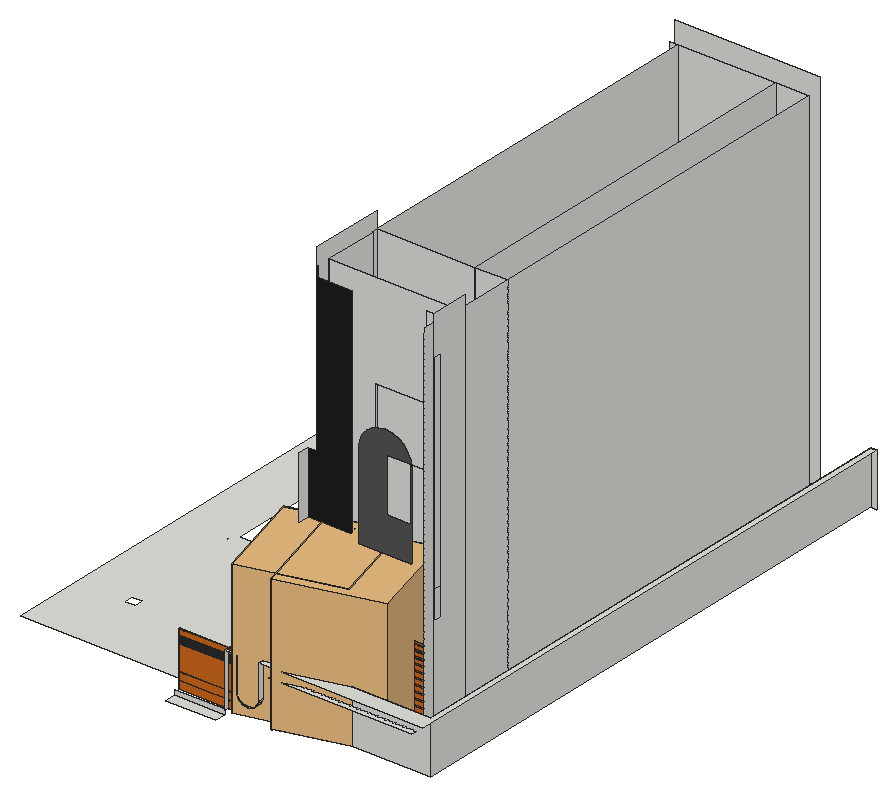
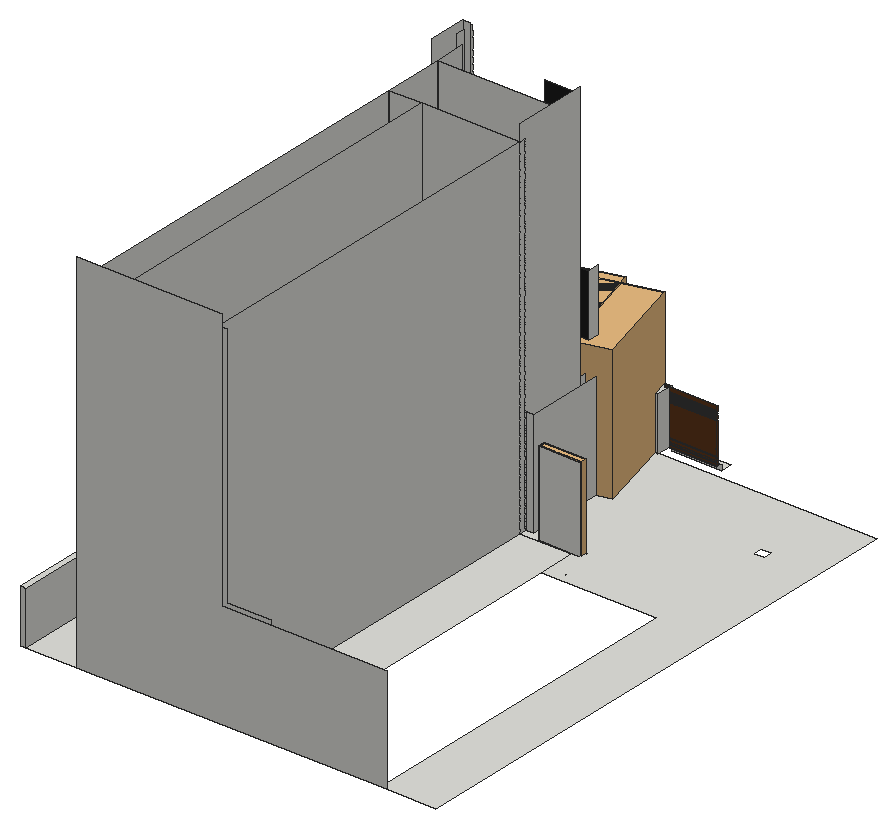
# SketchUp Ruby script. Lengths in inches.
U = 1.inch
M = Sketchup.active_model
def pt(a) = Geom::Point3d.new(a.map { |v| v * U })
def face(e, loops, mat)
  f = e.add_face(loops[0].map { |a| pt(a) })
  loops[1..].each { |l| e.add_face(l.map { |a| pt(a) }).erase! }
  f.material = f.back_material = mat if mat
  f
end
# faces: each face lists its corners as indices into pts; further lists are holes
def faces(e, pts, list, mat = nil) = list.each { |f| face(e, (f[0].is_a?(Array) ? f : [f]).map { |l| l.map { |i| pts[i] } }, mat) }
# xy, xz, yz: faces in a plane at the given z, y or x. An outline is a flat list of corners, or four numbers for a rectangle; further outlines are holes
def ring(l) = l.size == 4 ? [[l[0], l[1]], [l[2], l[1]], [l[2], l[3]], [l[0], l[3]]] : l.each_slice(2).to_a
def flat(e, list, mat, &to3) = list.each { |f| face(e, (f[0].is_a?(Array) ? f : [f]).map { |l| ring(l).map { |u, v| to3.(u, v) } }, mat) }
def xy(e, z, list, mat = nil) = flat(e, list, mat) { |x, y| [x, y, z] }
def xz(e, y, list, mat = nil) = flat(e, list, mat) { |x, z| [x, y, z] }
def yz(e, x, list, mat = nil) = flat(e, list, mat) { |y, z| [x, y, z] }
def lines(e, pts, list) = list.each { |a, b| e.add_line(pt(pts[a]), pt(pts[b])) }
# prism: a flat outline (further loops are holes) pulled along v
def prism(e, loops, v, mat = nil)
  f = face(e, loops, mat); d = Geom::Vector3d.new(v.map { |x| x * U })
  f.pushpull(f.normal.samedirection?(d) ? d.length : -d.length)
end
def box(e, o, s, mat = nil) = prism(e, [[o, [o[0] + s[0], o[1], o[2]], [o[0] + s[0], o[1] + s[1], o[2]], [o[0], o[1] + s[1], o[2]]]], [0, 0, s[2]], mat)
def at(x, y, z, deg = 0) = Geom::Transformation.translation(pt([x, y, z])) * Geom::Transformation.rotation(ORIGIN, Z_AXIS, deg.degrees)
def axes(o, x, y, z) = Geom::Transformation.new([*x, 0, *y, 0, *z, 0, *pt(o).to_a, 1])
def part(name) = M.definitions.add(name)
# library, detail: a bought-in or finely detailed component or shape, given as its bounding box
def library(name, o, s) = part(name).tap { |d| box(d.entities, o, s) }
def detail(e, o, s) = box(e.add_group.entities, o, s)
def put(e, d, t, mat = nil) = e.add_instance(d, t).tap { |i| i.material = mat if mat }
def group(e, t, mat = nil) = e.add_group.tap { |g| g.transformation = t; g.material = mat if mat }.entities
root = M.entities
M.materials.add("[0041_Chocolate]").color = [210, 105, 30]
M.materials.add("[Color M06]").color = [84, 84, 84]
M.materials.add("[Color M08]").color = [30, 30, 30]
M.materials.add("[Wood Veneer 01]2").color = [94, 55, 29]
c1 = library("元件\#5",[-4.39,0,0],[5.37,35.83,90.55])
c2 = part("Slatted screen panel")
xy(c2.entities,0,[[0,0,255.91,1.97]],"[Wood Veneer 01]2")
xy(c2.entities,16.54,[[0,1.18,255.91,1.97]],"[Wood Veneer 01]2")
xy(c2.entities,16.93,[[0,0,255.91,1.18]],"[Wood Veneer 01]2")
xy(c2.entities,17.78,[[0,0,255.91,1.18]],"[Wood Veneer 01]2")
xy(c2.entities,34.45,[[0,0,255.91,1.18]],"[Wood Veneer 01]2")
xy(c2.entities,35.07,[[0,0,255.91,1.18]],"[Wood Veneer 01]2")
xy(c2.entities,89.37,[[0,0,255.91,1.97]],"[Wood Veneer 01]2")
xy(c2.entities,92.91,[[0,0,255.91,1.97]],"[Wood Veneer 01]2")
xy(c2.entities,94.49,[[0,0,255.91,1.97]],"[Wood Veneer 01]2")
xy(c2.entities,97.64,[[0,0,255.91,1.97]],"[Wood Veneer 01]2")
xy(c2.entities,99.21,[[0,0,255.91,1.97]],"[Wood Veneer 01]2")
xy(c2.entities,102.36,[[0,0,255.91,1.97]],"[Wood Veneer 01]2")
xy(c2.entities,103.9375,[[0,0,255.91,1.97]],"[Wood Veneer 01]2")
xy(c2.entities,107.48,[[0,0,255.91,1.97]],"[Wood Veneer 01]2")
xy(c2.entities,119.29,[[0,0,255.91,1.97]],"[Wood Veneer 01]2")
xz(c2.entities,0,[[0,0,255.91,16.93],[0,17.78,255.91,34.45],[0,35.07,255.91,89.37],[0,92.91,255.91,94.49],[0,97.64,255.91,99.21],
  [0,102.36,255.91,103.9375],[0,107.48,255.91,119.29]],"[0041_Chocolate]")
xz(c2.entities,1.18,[[0,16.54,255.91,16.93],[0,16.93,255.91,17.78],[0,34.45,255.91,35.07]],"[Wood Veneer 01]2")
xz(c2.entities,1.97,[[0,0,255.91,1.57],[0,1.57,255.91,5.51],[0,5.51,255.91,7.09],[0,7.09,255.91,11.8125],[0,11.8125,255.91,16.54],
  [0,16.54,255.91,19.69],[0,19.69,255.91,89.37],[0,92.91,255.91,94.49],[0,97.64,255.91,99.21],[0,102.36,255.91,103.9375],
  [0,107.48,255.91,109.84],[0,109.84,255.91,119.29]],"[Wood Veneer 01]2")
yz(c2.entities,0,[[0,0,1.97,1.57],[0,1.57,1.97,5.51],[0,5.51,1.97,7.09],[0,7.09,1.97,11.8125],[0,11.8125,0,16.93,1.18,16.93,1.18,16.54,1.97,16.54,1.97,11.8125],
  [1.18,16.54,1.97,19.69],[0,17.78,0,34.45,1.18,34.45,1.18,35.07,0,35.07,0,89.37,1.97,89.37,1.97,19.69,1.18,19.69,1.18,17.78],[0,92.91,1.97,94.49],[0,97.64,1.97,99.21],[0,102.36,1.97,103.9375],
  [0,107.48,1.97,109.84],[0,109.84,1.97,119.29]],"[Wood Veneer 01]2")
yz(c2.entities,255.91,[[0,0,1.97,1.57],[0,1.57,1.97,5.51],[0,5.51,1.97,7.09],[0,7.09,1.97,11.8125],[0,11.8125,1.97,11.8125,1.97,16.54,1.18,16.54,1.18,16.93,0,16.93],
  [1.18,16.54,1.97,19.69],[0,17.78,1.18,17.78,1.18,19.69,1.97,19.69,1.97,89.37,0,89.37,0,35.07,1.18,35.07,1.18,34.45,0,34.45],[0,92.91,1.97,94.49],[0,97.64,1.97,99.21],[0,102.36,1.97,103.9375],
  [0,107.48,1.97,109.84],[0,109.84,1.97,119.29]],"[Wood Veneer 01]2")
p = [[255.91,1.97,103.9375],[255.91,1.97,107.48],[0,1.97,107.48],[0,1.97,103.9375],[0,1.97,92.91],[0,1.97,89.37],
  [255.91,1.97,99.21],[255.91,1.97,102.36],[255.91,1.97,89.37],[255.91,1.97,92.91],[0,1.97,97.64],[0,1.97,94.49],
  [0,1.97,102.36],[0,1.97,99.21],[255.91,1.97,94.49],[255.91,1.97,97.64],[240.94,0,5.51],[240.94,1.97,5.51]]
lines(c2.entities,p,[[0,1],[2,3],[4,5],[6,7],[8,9],[10,11],[12,13],[14,15],[16,17]])
c3 = library("Palm tree",[-4.09,-4.52,0],[193.52,193.51,258.93])
c4 = part("Palm+Tree")
put(c4.entities,c3,at(25.51,-21.81,0,15))
xy(root,0.73,[[2083.4,185.9375,2140.42,198.625]])
xy(root,6.125,[[[1894.57,217.125,2357.5,217.125,2357.5,838.14,1949.9,838.14,1949.9,439.98,2068.38,439.98,2068.38,397.86,2078.42,397.86,2078.42,405.05,2125.61,405.05,2125.61,397.86,2145.53,397.86,2145.53,406.38,2087.21,406.38,2087.21,448.51,1957.13,448.51,1957.13,830.91,2293.73,830.91,2293.73,336.27,2300.52,336.27,2300.52,292.45,2299.64,292.45,2299.64,280.47,2198.21,280.47,2198.21,292.45,2197.71,292.45,2197.71,305.58,2148.59,305.58,2148.59,292.45,2137,292.45,2137,397.86,2125.61,397.86,2125.61,405.05,2078.42,405.05,2078.42,397.86,2068.38,397.86,2068.38,439.98,1949.9,439.98,1949.9,838.14,1894.57,838.14],[1949.9,294.33,1962.9,305.58]],[2198.21,280.47,2293.73,280.47,2293.73,292.45,2292.85,292.45,2292.85,302.0625,2198.21,302.0625],[2293.73,280.47,2299.64,292.45],[2137,292.45,2148.59,305.58],[2197.71,292.45,2198.21,302.46],
  [2292.85,292.45,2293.73,302.46],[2293.73,292.45,2300.52,302.46],[2198.21,302.0625,2292.85,302.46],[[2198.21,302.46,2293.73,302.46,2293.73,406.38,2145.53,406.38,2145.53,397.86,2137,397.86,2137,305.58,2148.59,305.58,2148.59,312.8125,2158.24,312.8125,2158.24,305.58,2198.21,305.58],[2145.53,321.34,2146.71,397.86]],[2198.21,302.46,2198.21,305.58,2158.24,305.58,2158.24,312.8125,2146.71,312.8125,2146.71,336.27,2293.73,336.27,2293.73,302.46],
  [2198.21,302.46,2198.21,305.58,2158.24,305.58,2158.24,312.8125,2198.21,312.8125,2198.21,305.58,2293.73,305.58,2293.73,302.46],[2197.71,302.46,2198.21,305.58],[2293.73,302.46,2300.52,305.58],[2137,305.58,2148.59,312.8125],[2198.21,305.58,2198.21,312.8125,2146.71,312.8125,2146.71,336.27,2293.73,336.27,2293.73,305.58],
  [2148.59,305.58,2158.24,312.8125],[2293.73,305.58,2300.52,336.27],[2137,312.8125,2137,397.86,2145.53,397.86,2145.53,321.34,2146.71,321.34,2146.71,312.8125],[2145.53,321.34,2146.71,397.86],[2146.71,336.27,2293.73,337.5625],
  [2146.71,337.5625,2293.73,337.5625,2293.73,406.38,2145.53,406.38,2145.53,399.07,2146.71,399.07],[2145.53,397.86,2146.71,399.07],[2087.21,406.38,2145.53,830.91],[2145.53,406.38,2256.73,830.91],[2256.73,406.38,2293.73,830.91]])
xy(root,11.08,[[2198.21,280.47,2299.64,281.47]],"[0041_Chocolate]")
xy(root,13.1875,[[2198.21,280.47,2299.64,281.47]],"[0041_Chocolate]")
xy(root,18.14,[[2198.21,280.47,2299.64,281.47]],"[0041_Chocolate]")
xy(root,20.25,[[2198.21,280.47,2299.64,281.47]],"[0041_Chocolate]")
xy(root,25.2,[[2198.21,280.47,2299.64,281.47]],"[0041_Chocolate]")
xy(root,27.3125,[[2198.21,280.47,2299.64,281.47]],"[0041_Chocolate]")
xy(root,32.27,[[2198.21,280.47,2299.64,281.47]],"[0041_Chocolate]")
xy(root,34.375,[[2198.21,280.47,2299.64,281.47]],"[0041_Chocolate]")
xy(root,39.33,[[2198.21,280.47,2299.64,281.47]],"[0041_Chocolate]")
xy(root,41.4375,[[2198.21,280.47,2299.64,281.47]],"[0041_Chocolate]")
xy(root,46.39,[[2198.21,280.47,2299.64,281.47]],"[0041_Chocolate]")
xy(root,48.5,[[2198.21,280.47,2299.64,281.47]],"[0041_Chocolate]")
xy(root,53.45,[[2198.21,280.47,2299.64,281.47]],"[0041_Chocolate]")
xy(root,55.1875,[[2189.5,198.625,2189.5,203.875,2191.125,203.875,2191.125,204.875,2191.875,204.875,2191.875,203.875,2195.125,203.875,2195.125,204.875,2195.875,204.875,2195.875,203.875,2199.125,203.875,2199.125,204.875,2199.875,204.875,2199.875,203.875,2203.125,203.875,2203.125,204.875,2203.875,204.875,2203.875,203.875,2207.125,203.875,2207.125,204.875,2207.875,204.875,2207.875,203.875,2211.125,203.875,2211.125,204.875,2211.875,204.875,2211.875,203.875,2215.125,203.875,2215.125,204.875,2215.875,204.875,2215.875,203.875,2219.125,203.875,2219.125,204.875,2219.875,204.875,2219.875,203.875,2223.125,203.875,2223.125,204.875,2223.875,204.875,2223.875,203.875,2227.125,203.875,2227.125,204.875,2227.875,204.875,2227.875,203.875,2231.125,203.875,2231.125,204.875,2231.875,204.875,2231.875,203.875,2235.125,203.875,2235.125,204.875,2235.875,204.875,2235.875,203.875,2239.125,203.875,2239.125,204.875,2239.875,204.875,2239.875,203.875,2243.125,203.875,2243.125,204.875,2243.875,204.875,2243.875,203.875,2247.125,203.875,2247.125,204.875,2247.875,204.875,2247.875,203.875,2251.125,203.875,2251.125,204.875,2251.875,204.875,2251.875,203.875,2255.125,203.875,2255.125,204.875,2255.875,204.875,2255.875,203.875,2259.125,203.875,2259.125,204.875,2259.875,204.875,2259.875,203.875,2263.125,203.875,2263.125,204.875,2263.875,204.875,2263.875,203.875,2267.125,203.875,2267.125,204.875,2267.875,204.875,2267.875,203.875,2271.125,203.875,2271.125,204.875,2271.875,204.875,2271.875,203.875,2275.125,203.875,2275.125,204.875,2275.875,204.875,2275.875,203.875,2279.125,203.875,2279.125,204.875,2279.875,204.875,2279.875,203.875,2283.125,203.875,2283.125,204.875,2283.875,204.875,2283.875,203.875,2287.125,203.875,2287.125,204.875,2287.875,204.875,2287.875,203.875,2291.125,203.875,2291.125,204.875,2291.875,204.875,2291.875,203.875,2295.125,203.875,2295.125,204.875,2295.875,204.875,2295.875,203.875,2299.125,203.875,2299.125,204.875,2299.875,204.875,2299.875,203.875,2303.125,203.875,2303.125,204.875,2303.875,204.875,2303.875,203.875,2307.125,203.875,2307.125,204.875,2307.875,204.875,2307.875,203.875,2311.125,203.875,2311.125,204.875,2311.875,204.875,2311.875,203.875,2315.125,203.875,2315.125,204.875,2315.875,204.875,2315.875,203.875,2319.125,203.875,2319.125,204.875,2319.875,204.875,2319.875,203.875,2323.125,203.875,2323.125,204.875,2323.875,204.875,2323.875,203.875,2327.125,203.875,2327.125,204.875,2327.875,204.875,2327.875,203.875,2331.125,203.875,2331.125,204.875,2331.875,204.875,2331.875,203.875,2335.125,203.875,2335.125,204.875,2335.875,204.875,2335.875,203.875,2339.125,203.875,2339.125,204.875,2339.875,204.875,2339.875,203.875,2343.125,203.875,2343.125,204.875,2343.875,204.875,2343.875,203.875,2347.125,203.875,2347.125,204.875,2347.875,204.875,2347.875,203.875,2351.125,203.875,2351.125,198.625]])
xy(root,55.5625,[[2198.21,280.47,2299.64,281.47]],"[0041_Chocolate]")
xy(root,60.52,[[2198.21,280.47,2299.64,281.47]],"[0041_Chocolate]")
xy(root,62.625,[[2198.21,280.47,2299.64,281.47]],"[0041_Chocolate]")
xy(root,66.125,[[2140.66,198.625,2153.79,198.625,2153.79,204.875,2178.1,204.875,2178.1,198.625,2364.02,198.625,2364.02,838.14,2357.5,838.14,2357.5,217.125,2140.66,217.125]])
xy(root,67.58,[[2198.21,280.47,2299.64,281.47]],"[0041_Chocolate]")
xy(root,69.6875,[[2198.21,280.47,2299.64,281.47]],"[0041_Chocolate]")
xy(root,74.64,[[2198.21,280.47,2234.41,281.47],[2252.36,280.47,2299.64,281.47]],"[0041_Chocolate]")
xy(root,76.75,[[2198.21,280.47,2229.32,281.47],[2257.45,280.47,2299.64,281.47]],"[0041_Chocolate]")
xy(root,81.7,[[2198.21,280.47,2222.48,281.47],[2264.29,280.47,2299.64,281.47]],"[0041_Chocolate]")
xy(root,83.8125,[[2198.21,280.47,2220.8,281.47],[2265.97,280.47,2299.64,281.47]],"[0041_Chocolate]")
xy(root,88.77,[[2198.21,280.47,2217.27,281.47],[2269.5,280.47,2299.64,281.47]],"[0041_Chocolate]")
xz(root,198.625,[[2083.4,0.73,2140.42,6.125]])
xz(root,204.875,[[2187.875,0,2189.5,55.1875]])
xz(root,204.875,[[2165.94,16.91,2168.74,17.23,2171.4,18.17,2173.77,19.69,2175.74,21.71,2177.21,24.11,2178.1,26.79,2178.1,66.125,2153.79,66.125,2153.79,26.79,2154.67,24.11,2156.14,21.71,2158.11,19.69,2160.49,18.17,2163.14,17.23]],"[0041_Chocolate]")
xz(root,217.125,[[2140.66,6.125,2357.5,66.125]])
xz(root,280.47,[[2198.21,6.125,2299.64,11.08],[2198.21,13.1875,2299.64,18.14],[2198.21,20.25,2299.64,25.2],[2198.21,27.3125,2299.64,32.27],[2198.21,34.375,2299.64,39.33],
  [2198.21,41.4375,2299.64,46.39],[2198.21,48.5,2299.64,53.45],[2198.21,55.5625,2299.64,60.52],[2198.21,62.625,2299.64,67.58],[2198.21,69.6875,2299.64,69.6875,2299.64,74.64,2252.36,74.64,2251.09,74.12,2243.38,73.1,2235.67,74.12,2234.41,74.64,2198.21,74.64],
  [2198.21,76.75,2229.32,76.75,2228.49,77.09,2222.48,81.7,2198.21,81.7],[2257.45,76.75,2299.64,76.75,2299.64,81.7,2264.29,81.7,2258.28,77.09],[2198.21,83.8125,2220.8,83.8125,2217.59,88,2217.27,88.77,2198.21,88.77],[2265.97,83.8125,2299.64,83.8125,2299.64,88.77,2269.5,88.77,2269.18,88]],"[0041_Chocolate]")
xz(root,281.47,[[2198.21,11.08,2299.64,13.1875],[2198.21,18.14,2299.64,20.25],[2198.21,25.2,2299.64,27.3125],[2198.21,32.27,2299.64,34.375],[2198.21,39.33,2299.64,41.4375],
  [2198.21,46.39,2299.64,48.5],[2198.21,53.45,2299.64,55.5625],[2198.21,60.52,2299.64,62.625],[2198.21,67.58,2299.64,69.6875],[2198.21,74.64,2234.41,74.64,2229.32,76.75,2198.21,76.75],
  [2252.36,74.64,2299.64,74.64,2299.64,76.75,2257.45,76.75],[2198.21,81.7,2222.48,81.7,2222.32,81.83,2220.8,83.8125,2198.21,83.8125],[2264.29,81.7,2299.64,81.7,2299.64,83.8125,2265.97,83.8125,2264.45,81.83],[2198.21,88.77,2217.27,88.77,2216.39,90.875,2198.21,90.875],[2269.5,88.77,2299.64,88.77,2299.64,90.875,2270.37,90.875]],"[0041_Chocolate]")
xz(root,292.45,[[2137,6.125,2148.59,132.47],[2292.85,6.125,2293.73,126.125],[2293.73,6.125,2299.64,126.125],[2299.64,6.125,2300.52,6.125,2300.52,421.25,2293.73,421.25,2293.73,141.26,2299.64,141.26]])
xz(root,295.65,[[[2243.38,73.1,2251.09,74.12,2252.36,74.64,2257.45,76.75,2258.28,77.09,2264.29,81.7,2264.45,81.83,2265.97,83.8125,2269.18,88,2269.5,88.77,2270.37,90.875,2272.16,95.18,2272.24,95.83,2272.43,97.27,2247.98,97.27,2247.98,145.27,2273.17,145.27,2273.17,253.3125,2272.52,258.27,2272.24,260.375,2272.16,261.02,2270.37,265.33,2269.5,267.4375,2269.18,268.21,2265.97,272.39,2264.45,274.375,2264.29,274.5,2258.28,279.11,2257.45,279.45,2252.36,281.5625,2251.09,282.09,2243.38,283.1,2235.67,282.09,2234.41,281.5625,2229.32,279.45,2228.49,279.11,2222.48,274.5,2222.32,274.375,2220.8,272.39,2217.59,268.21,2217.27,267.4375,2216.39,265.33,2214.61,261.02,2214.53,260.375,2214.25,258.27,2213.6,253.3125,2213.6,102.89,2214.25,97.9375,2214.53,95.83,2214.61,95.18,2216.39,90.875,2217.27,88.77,2217.59,88,2220.8,83.8125,2222.32,81.83,2222.48,81.7,2228.49,77.09,2229.32,76.75,2234.41,74.64,2235.67,74.12],[2245.83,196.89,2272.52,258.27]]],"[Color M06]")
xz(root,302.46,[[2197.71,6.125,2198.21,8.32],[2198.21,6.125,2285.18,8.32],[2285.18,6.125,2292.85,8.32],[2292.85,6.125,2293.73,8.32],[2293.73,6.125,2300.52,8.32],
  [2197.71,8.32,2198.21,95.62],[2198.21,8.32,2285.18,126.125],[2285.18,8.32,2292.85,109.9375],[2292.85,8.32,2293.73,109.9375]])
xz(root,305.58,[[2148.59,6.125,2197.71,6.125,2197.71,126.125,2198.21,126.125,2198.21,402.64,2158.24,402.64,2158.24,226.8,2148.59,226.8]],"[Color M08]")
xz(root,312.8125,[[2146.71,6.125,2148.59,126.125],[2148.59,6.125,2158.24,126.125]])
xz(root,321.34,[[2145.53,6.125,2146.71,402.64]])
xz(root,337.5625,[[[2146.71,6.125,2293.73,402.64],[2198.21,226.8,2291.02,295.72]]])
xz(root,397.86,[[2137,6.125,2146.71,126.125]])
xz(root,399.07,[[2145.53,6.125,2146.71,402.64]])
xz(root,405.05,[[2078.42,6.125,2125.61,101.1875]])
xz(root,406.38,[[2145.53,6.125,2256.73,402.64],[2256.73,6.125,2293.73,402.64]])
xz(root,830.91,[[2087.21,6.125,2087.21,126.125,2137,126.125,2137,402.64,2145.53,402.64,2145.53,6.125],[2145.53,6.125,2256.73,402.64],[2256.73,6.125,2293.73,402.64]])
xz(root,838.14,[[1949.9,6.125,1949.9,126.125,2137,126.125,2137,421.25,2300.52,421.25,2300.52,6.125],[2357.5,6.125,2364.02,66.125]])
yz(root,2125.61,[[397.86,6.125,405.05,101.1875]])
yz(root,2137,[[292.45,6.125,292.45,132.47,305.58,132.47,305.58,126.125,397.86,126.125,397.86,6.125]])
yz(root,2140.66,[[198.625,6.125,217.125,66.125]])
yz(root,2145.53,[[321.34,6.125,321.34,421.25,406.38,421.25,406.38,402.64,399.07,402.64,399.07,6.125],[399.07,6.125,406.38,402.64],[406.38,6.125,830.91,402.64]])
yz(root,2146.71,[[312.8125,6.125,321.34,126.125],[321.34,6.125,336.27,126.125],[336.27,6.125,337.5625,126.125],[337.5625,6.125,397.86,126.125],[397.86,6.125,399.07,6.125,399.07,402.64,337.5625,402.64,337.5625,126.125,397.86,126.125]])
yz(root,2148.59,[[292.45,6.125,305.58,226.8]])
yz(root,2153.79,[[198.625,26.79,204.875,66.125]])
yz(root,2178.1,[[198.625,26.79,204.875,66.125]])
yz(root,2189.5,[[203.875,0,204.875,55.1875]])
yz(root,2197.71,[[302.46,6.125,305.58,8.32],[302.46,8.32,305.58,95.62]])
yz(root,2198.21,[[280.47,6.125,280.47,11.08,281.47,11.08,281.47,13.1875,280.47,13.1875,280.47,18.14,281.47,18.14,281.47,20.25,280.47,20.25,280.47,25.2,281.47,25.2,281.47,27.3125,280.47,27.3125,280.47,32.27,281.47,32.27,281.47,34.375,280.47,34.375,280.47,39.33,281.47,39.33,281.47,41.4375,280.47,41.4375,280.47,46.39,281.47,46.39,281.47,48.5,280.47,48.5,280.47,53.45,281.47,53.45,281.47,55.5625,280.47,55.5625,280.47,60.52,281.47,60.52,281.47,62.625,280.47,62.625,280.47,67.58,281.47,67.58,281.47,69.6875,280.47,69.6875,280.47,74.64,281.47,74.64,281.47,76.75,280.47,76.75,280.47,81.7,281.47,81.7,281.47,83.8125,280.47,83.8125,280.47,88.77,281.47,88.77,281.47,90.875,280.47,90.875,280.47,95.83,281.47,95.83,281.47,97.9375,280.47,97.9375,280.47,102.89,281.47,102.89,281.47,105,280.47,105,280.47,109.95,281.47,109.95,281.47,112.0625,280.47,112.0625,280.47,117.02,281.47,117.02,281.47,119.125,280.47,119.125,280.47,124.08,281.47,124.08,281.47,126.1875,280.47,126.1875,280.47,131.14,281.47,131.14,281.47,133.25,280.47,133.25,280.47,138.2,281.47,138.2,281.47,140.3125,280.47,140.3125,280.47,141.26,292.45,141.26,292.45,126.125,302.46,126.125,302.46,6.125]])
yz(root,2256.73,[[406.38,6.125,830.91,402.64]])
yz(root,2292.85,[[292.45,6.125,302.46,126.125]])
yz(root,2293.73,[[302.46,6.125,337.5625,402.64],[337.5625,6.125,406.38,402.64],[406.38,6.125,830.91,402.64]])
yz(root,2299.64,[[280.47,6.125,292.45,6.125,292.45,141.26,302.46,141.26,302.46,411.82,281.47,411.82,281.47,405.64,280.47,405.64,280.47,400.6875,281.47,400.6875,281.47,398.77,280.47,398.77,280.47,393.8125,281.47,393.8125,281.47,391.89,280.47,391.89,280.47,386.9375,281.47,386.9375,281.47,385.02,280.47,385.02,280.47,380.0625,281.47,380.0625,281.47,378.14,280.47,378.14,280.47,373.1875,281.47,373.1875,281.47,371.27,280.47,371.27,280.47,366.3125,281.47,366.3125,281.47,364.2,280.47,364.2,280.47,359.25,281.47,359.25,281.47,357.14,280.47,357.14,280.47,352.1875,281.47,352.1875,281.47,350.08,280.47,350.08,280.47,345.125,281.47,345.125,281.47,343.02,280.47,343.02,280.47,338.0625,281.47,338.0625,281.47,335.95,280.47,335.95,280.47,331,281.47,331,281.47,328.89,280.47,328.89,280.47,323.9375,281.47,323.9375,281.47,321.83,280.47,321.83,280.47,316.875,281.47,316.875,281.47,314.77,280.47,314.77,280.47,309.8125,281.47,309.8125,281.47,307.7,280.47,307.7,280.47,302.75,281.47,302.75,281.47,300.64,280.47,300.64,280.47,295.6875,281.47,295.6875,281.47,293.58,280.47,293.58,280.47,288.625,281.47,288.625,281.47,286.52,280.47,286.52,280.47,281.5625,281.47,281.5625,281.47,279.45,280.47,279.45,280.47,274.5,281.47,274.5,281.47,272.39,280.47,272.39,280.47,267.4375,281.47,267.4375,281.47,265.33,280.47,265.33,280.47,260.375,281.47,260.375,281.47,258.27,280.47,258.27,280.47,253.3125,281.47,253.3125,281.47,251.2,280.47,251.2,280.47,246.25,281.47,246.25,281.47,244.14,280.47,244.14,280.47,239.1875,281.47,239.1875,281.47,237.08,280.47,237.08,280.47,232.125,281.47,232.125,281.47,230.02,280.47,230.02,280.47,225.0625,281.47,225.0625,281.47,222.95,280.47,222.95,280.47,218,281.47,218,281.47,215.89,280.47,215.89,280.47,210.9375,281.47,210.9375,281.47,208.83,280.47,208.83,280.47,203.875,281.47,203.875,281.47,201.77,280.47,201.77,280.47,196.8125,281.47,196.8125,281.47,194.7,280.47,194.7,280.47,189.75,281.47,189.75,281.47,187.64,280.47,187.64,280.47,182.6875,281.47,182.6875,281.47,180.58,280.47,180.58,280.47,175.625,281.47,175.625,281.47,173.52,280.47,173.52,280.47,168.5625,281.47,168.5625,281.47,166.45,280.47,166.45,280.47,161.5,281.47,161.5,281.47,159.39,280.47,159.39,280.47,154.4375,281.47,154.4375,281.47,152.33,280.47,152.33,280.47,147.375,281.47,147.375,281.47,145.27,280.47,145.27,280.47,140.3125,281.47,140.3125,281.47,138.2,280.47,138.2,280.47,133.25,281.47,133.25,281.47,131.14,280.47,131.14,280.47,126.1875,281.47,126.1875,281.47,124.08,280.47,124.08,280.47,119.125,281.47,119.125,281.47,117.02,280.47,117.02,280.47,112.0625,281.47,112.0625,281.47,109.95,280.47,109.95,280.47,105,281.47,105,281.47,102.89,280.47,102.89,280.47,97.9375,281.47,97.9375,281.47,95.83,280.47,95.83,280.47,90.875,281.47,90.875,281.47,88.77,280.47,88.77,280.47,83.8125,281.47,83.8125,281.47,81.7,280.47,81.7,280.47,76.75,281.47,76.75,281.47,74.64,280.47,74.64,280.47,69.6875,281.47,69.6875,281.47,67.58,280.47,67.58,280.47,62.625,281.47,62.625,281.47,60.52,280.47,60.52,280.47,55.5625,281.47,55.5625,281.47,53.45,280.47,53.45,280.47,48.5,281.47,48.5,281.47,46.39,280.47,46.39,280.47,41.4375,281.47,41.4375,281.47,39.33,280.47,39.33,280.47,34.375,281.47,34.375,281.47,32.27,280.47,32.27,280.47,27.3125,281.47,27.3125,281.47,25.2,280.47,25.2,280.47,20.25,281.47,20.25,281.47,18.14,280.47,18.14,280.47,13.1875,281.47,13.1875,281.47,11.08,280.47,11.08]])
yz(root,2300.52,[[292.45,6.125,336.27,6.125,336.27,421.25,292.45,421.25,292.45,376.875,302.46,376.875,302.46,109.9375,299.11,109.9375,295.02,110.21,292.45,110.72]])
yz(root,2357.5,[[217.125,6.125,838.14,66.125]])
p = [[2165.94,204.875,16.91],[2163.14,204.875,17.23],[2163.14,198.625,17.23],[2165.94,198.625,16.91],[2168.74,204.875,17.23],[2168.74,198.625,17.23],
  [2160.49,204.875,18.17],[2160.49,198.625,18.17],[2171.4,204.875,18.17],[2171.4,198.625,18.17],[2158.11,204.875,19.69],[2158.11,198.625,19.69],
  [2173.77,204.875,19.69],[2173.77,198.625,19.69],[2156.14,204.875,21.71],[2156.14,198.625,21.71],[2175.74,204.875,21.71],[2175.74,198.625,21.71],
  [2154.67,204.875,24.11],[2154.67,198.625,24.11],[2177.21,204.875,24.11],[2177.21,198.625,24.11],[2153.79,204.875,26.79],[2153.79,198.625,26.79],
  [2178.1,204.875,26.79],[2178.1,198.625,26.79],[2235.67,295.65,74.12],[2235.67,280.47,74.12],[2243.38,280.47,73.1],[2243.38,295.65,73.1],
  [2251.09,280.47,74.12],[2251.09,295.65,74.12],[2234.41,295.65,74.64],[2234.41,281.47,74.64],[2234.41,280.47,74.64],[2252.36,280.47,74.64],
  [2252.36,281.47,74.64],[2252.36,295.65,74.64],[2229.32,281.47,76.75],[2229.32,295.65,76.75],[2257.45,281.47,76.75],[2257.45,295.65,76.75],
  [2228.49,295.65,77.09],[2228.49,280.47,77.09],[2229.32,280.47,76.75],[2257.45,280.47,76.75],[2258.28,280.47,77.09],[2258.28,295.65,77.09],
  [2222.48,295.65,81.7],[2222.48,281.47,81.7],[2222.48,280.47,81.7],[2264.29,280.47,81.7],[2264.29,281.47,81.7],[2264.29,295.65,81.7],
  [2222.32,281.47,81.83],[2222.32,295.65,81.83],[2264.45,281.47,81.83],[2264.45,295.65,81.83],[2220.8,281.47,83.8125],[2220.8,295.65,83.8125],
  [2265.97,281.47,83.8125],[2265.97,295.65,83.8125],[2217.59,295.65,88],[2217.59,280.47,88],[2220.8,280.47,83.8125],[2265.97,280.47,83.8125],
  [2269.18,280.47,88],[2269.18,295.65,88],[2217.27,295.65,88.77],[2217.27,281.47,88.77],[2217.27,280.47,88.77],[2269.5,280.47,88.77],
  [2269.5,281.47,88.77],[2269.5,295.65,88.77],[2216.39,281.47,90.875],[2216.39,295.65,90.875],[2270.37,281.47,90.875],[2270.37,295.65,90.875],
  [2198.21,312.8125,24.125],[2198.21,312.8125,6.125],[2198.21,321.34,24.125]]
faces(root,p,[[0,1,2,3],[4,0,3,5],[1,6,7,2],[8,4,5,9],[6,10,11,7],[12,8,9,13],[10,14,15,11],[16,12,13,17],
  [14,18,19,15],[20,16,17,21],[18,22,23,19],[24,20,21,25]])
faces(root,p,[[26,27,28,29],[29,28,30,31],[32,33,34,27,26],[31,30,35,36,37],[38,33,32,39],[36,40,41,37],[42,43,44,38,39],[41,40,45,46,47],
  [48,49,50,43,42],[47,46,51,52,53],[54,49,48,55],[52,56,57,53],[58,54,55,59],[56,60,61,57],[62,63,64,58,59],[61,60,65,66,67],
  [68,69,70,63,62],[67,66,71,72,73],[74,69,68,75],[72,76,77,73]],"[Color M06]")
lines(root,p,[[78,79],[78,80]])
put(root,c1,axes([2078.42,398.25,6.11],[0,-1.05,0],[1.302,0,0],[0,0,1.05]))
put(root,c2,axes([2085.49,201.88,6.125],[0.23355,0,0],[0,0.5124,0],[0,0,0.5124]),"[0041_Chocolate]")
put(root,c4,axes([2136.29,212.94,6.125],[0.58344,0,0],[0,0.58344,0],[0,0,0.58344]),"[Color M06]")
put(root,c4,axes([2180.11,212.94,6.125],[0.58344,0,0],[0,0.58344,0],[0,0,0.58344]),"[Color M06]")
